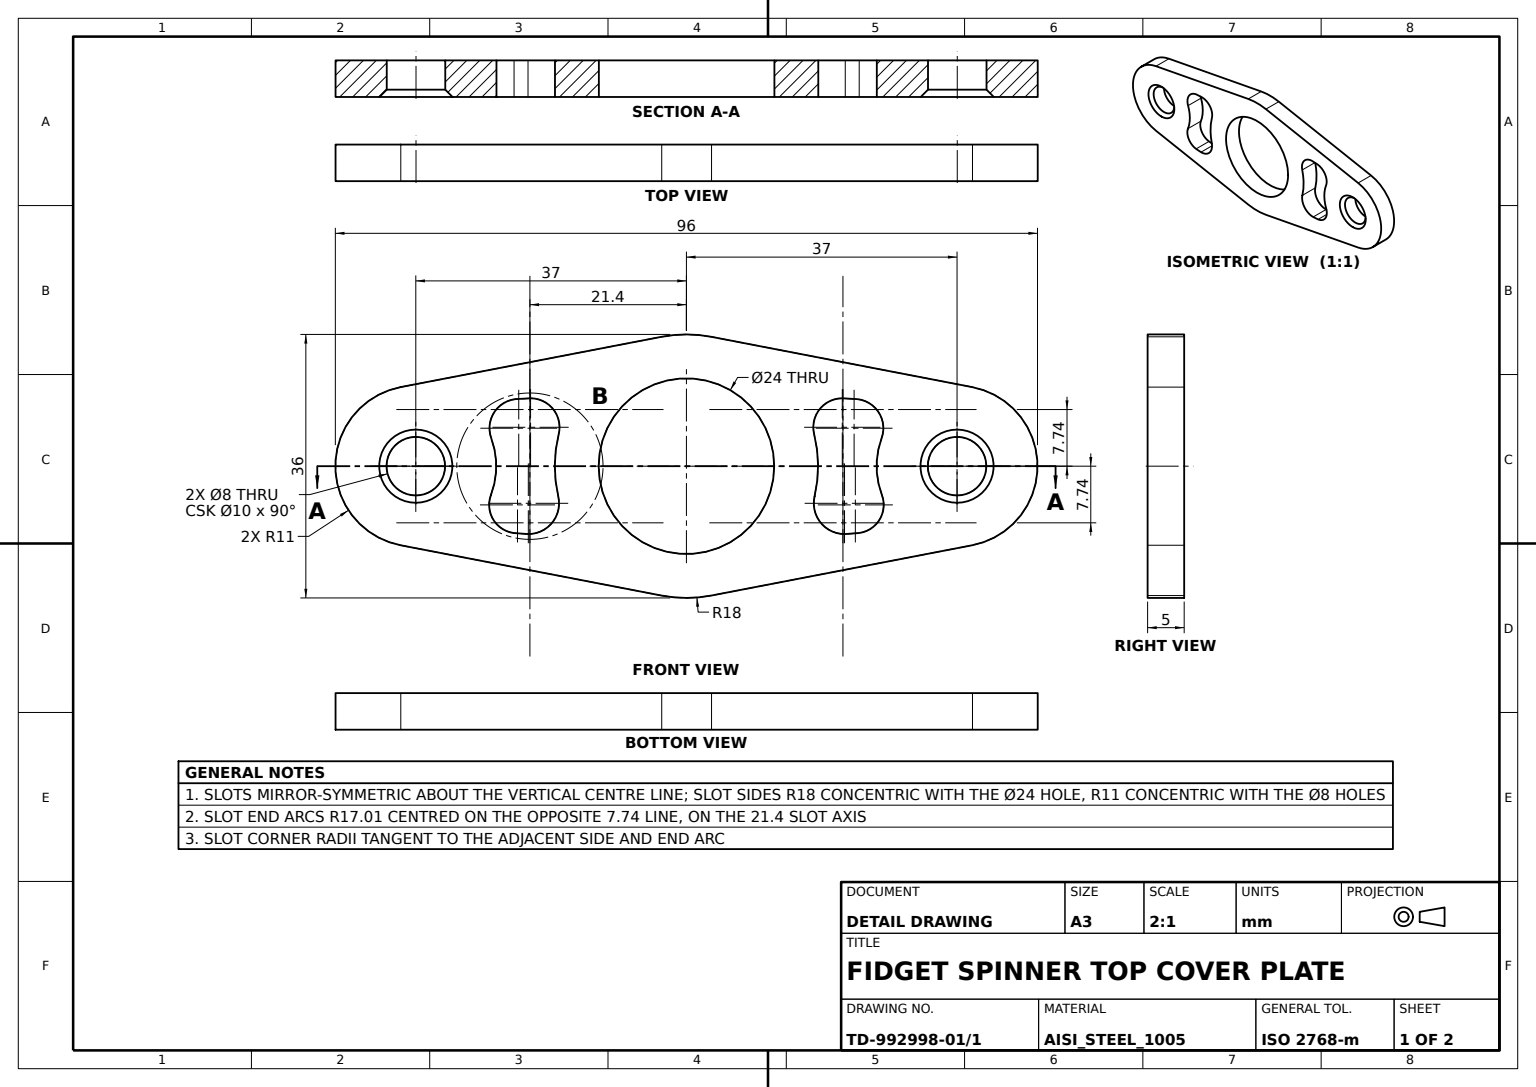
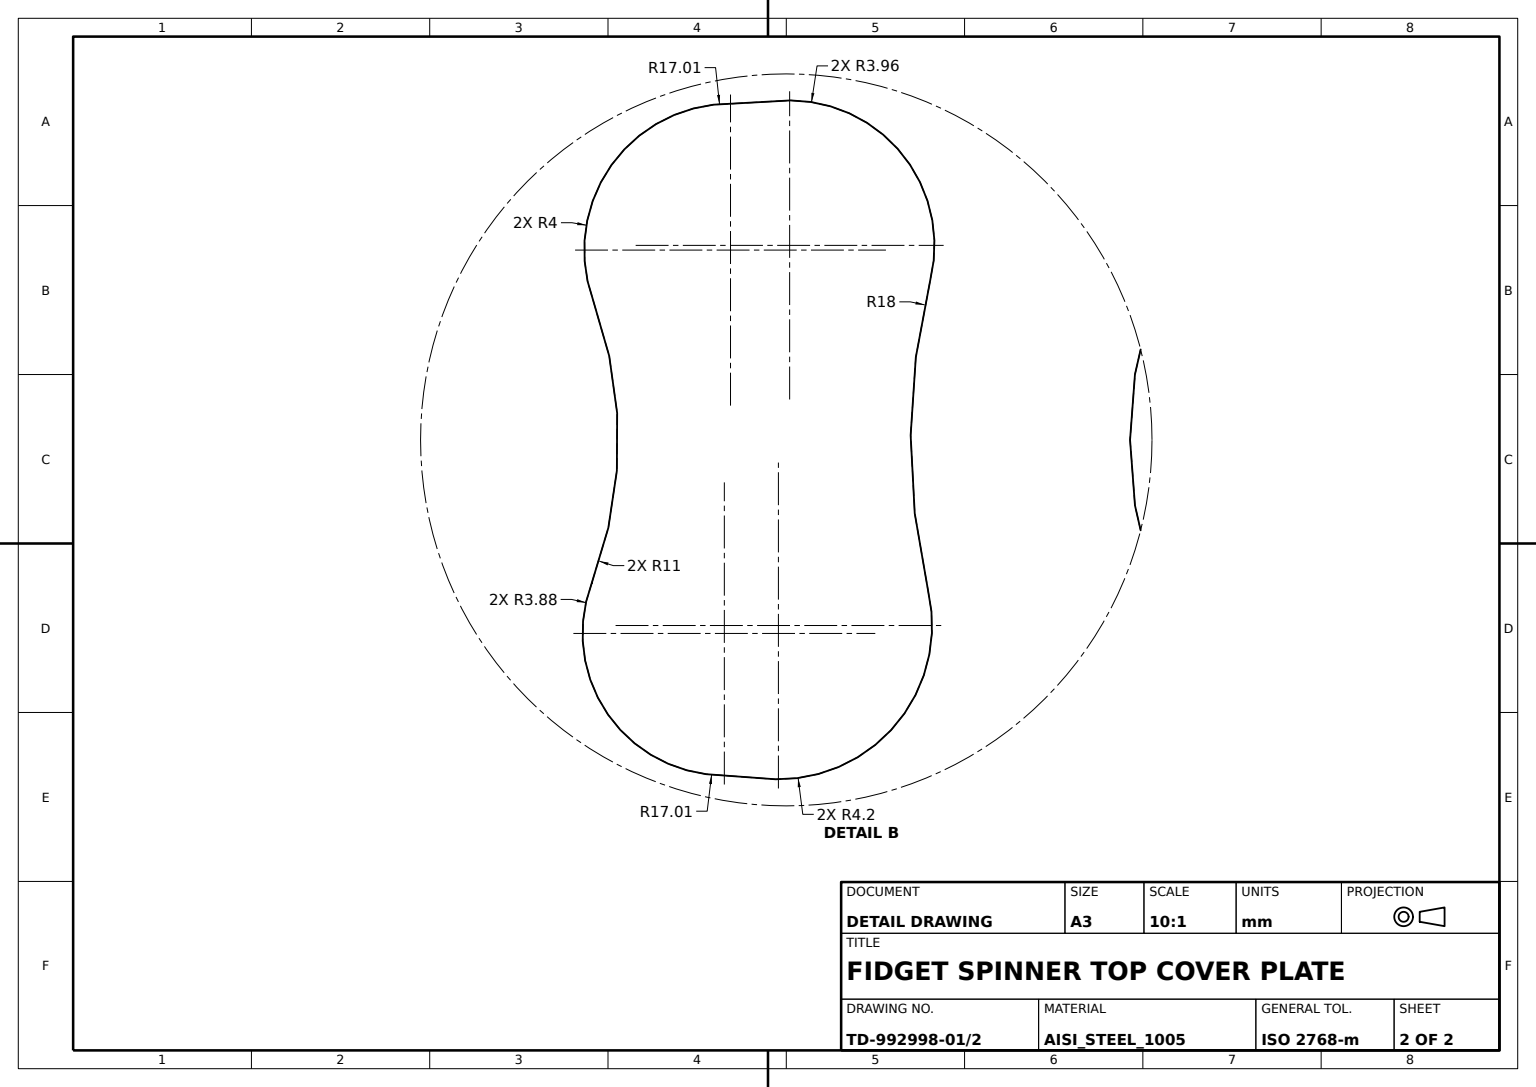
ISO-10303-21;
HEADER;
FILE_DESCRIPTION((''),'2;1');
FILE_NAME('','',(''),(''),'','','');
FILE_SCHEMA(('AUTOMOTIVE_DESIGN'));
ENDSEC;
DATA;
#1=APPLICATION_CONTEXT('');
#2=PRODUCT_CONTEXT('',#1,'mechanical');
#3=PRODUCT('','','',(#2));
#4=PRODUCT_DEFINITION_FORMATION('','',#3);
#5=PRODUCT_DEFINITION_CONTEXT('',#1,'design');
#6=PRODUCT_DEFINITION('','',#4,#5);
#7=PRODUCT_DEFINITION_SHAPE('','',#6);
#8=(LENGTH_UNIT()NAMED_UNIT(*)SI_UNIT(.MILLI.,.METRE.));
#9=(NAMED_UNIT(*)PLANE_ANGLE_UNIT()SI_UNIT($,.RADIAN.));
#10=(NAMED_UNIT(*)SI_UNIT($,.STERADIAN.)SOLID_ANGLE_UNIT());
#11=UNCERTAINTY_MEASURE_WITH_UNIT(LENGTH_MEASURE(0.005),#8,'distance_accuracy_value','');
#12=(GEOMETRIC_REPRESENTATION_CONTEXT(3)GLOBAL_UNCERTAINTY_ASSIGNED_CONTEXT((#11))GLOBAL_UNIT_ASSIGNED_CONTEXT((#8,#9,#10))REPRESENTATION_CONTEXT('',''));
#13=CARTESIAN_POINT('',(3.405405,-5.,17.674932));
#14=VERTEX_POINT('',#13);
#15=CARTESIAN_POINT('',(3.405405,0.,17.674932));
#16=VERTEX_POINT('',#15);
#17=DIRECTION('',(0.,1.,0.));
#18=VECTOR('',#17,1000.);
#19=LINE('',#13,#18);
#20=EDGE_CURVE('',#14,#16,#19,.T.);
#21=ORIENTED_EDGE('',*,*,#20,.T.);
#22=CARTESIAN_POINT('',(-3.405405,0.,17.674932));
#23=VERTEX_POINT('',#22);
#24=CARTESIAN_POINT('',(0.,0.,0.));
#25=DIRECTION('',(0.,-1.,0.));
#26=DIRECTION('',(1.,0.,0.));
#27=AXIS2_PLACEMENT_3D('',#24,#25,#26);
#28=CIRCLE('',#27,18.);
#29=EDGE_CURVE('',#16,#23,#28,.T.);
#30=ORIENTED_EDGE('',*,*,#29,.T.);
#31=CARTESIAN_POINT('',(-3.405405,-5.,17.674932));
#32=VERTEX_POINT('',#31);
#33=LINE('',#31,#18);
#34=EDGE_CURVE('',#32,#23,#33,.T.);
#35=ORIENTED_EDGE('',*,*,#34,.F.);
#36=CARTESIAN_POINT('',(0.,-5.,0.));
#37=AXIS2_PLACEMENT_3D('',#36,#25,#26);
#38=CIRCLE('',#37,18.);
#39=EDGE_CURVE('',#14,#32,#38,.T.);
#40=ORIENTED_EDGE('',*,*,#39,.F.);
#41=EDGE_LOOP('',(#21,#30,#35,#40));
#42=FACE_BOUND('',#41,.T.);
#43=DIRECTION('',(0.,0.,1.));
#44=AXIS2_PLACEMENT_3D('',#36,#17,#43);
#45=CYLINDRICAL_SURFACE('',#44,18.);
#46=ADVANCED_FACE('',(#42),#45,.T.);
#47=CARTESIAN_POINT('',(-33.,0.,0.));
#48=VERTEX_POINT('',#47);
#49=CARTESIAN_POINT('',(-37.,0.,0.));
#50=AXIS2_PLACEMENT_3D('',#49,#25,#26);
#51=CIRCLE('',#50,4.);
#52=EDGE_CURVE('',#48,#48,#51,.T.);
#53=ORIENTED_EDGE('',*,*,#52,.F.);
#54=EDGE_LOOP('',(#53));
#55=FACE_BOUND('',#54,.T.);
#56=CARTESIAN_POINT('',(-37.,-4.,-4.));
#57=VERTEX_POINT('',#56);
#58=CARTESIAN_POINT('',(-37.,-4.,0.));
#59=DIRECTION('',(0.,0.,-1.));
#60=AXIS2_PLACEMENT_3D('',#58,#25,#59);
#61=CIRCLE('',#60,4.);
#62=EDGE_CURVE('',#57,#57,#61,.T.);
#63=ORIENTED_EDGE('',*,*,#62,.T.);
#64=EDGE_LOOP('',(#63));
#65=FACE_BOUND('',#64,.T.);
#66=CARTESIAN_POINT('',(-37.,-5.,0.));
#67=AXIS2_PLACEMENT_3D('',#66,#17,#43);
#68=CYLINDRICAL_SURFACE('',#67,4.);
#69=ADVANCED_FACE('',(#55,#65),#68,.F.);
#70=CARTESIAN_POINT('',(39.081081,0.,10.801347));
#71=VERTEX_POINT('',#70);
#72=DIRECTION('',(-0.981940655,0.,0.189189189));
#73=VECTOR('',#72,1000.);
#74=LINE('',#70,#73);
#75=EDGE_CURVE('',#71,#16,#74,.T.);
#76=ORIENTED_EDGE('',*,*,#75,.T.);
#77=ORIENTED_EDGE('',*,*,#20,.F.);
#78=CARTESIAN_POINT('',(39.081081,-5.,10.801347));
#79=VERTEX_POINT('',#78);
#80=LINE('',#78,#73);
#81=EDGE_CURVE('',#79,#14,#80,.T.);
#82=ORIENTED_EDGE('',*,*,#81,.F.);
#83=LINE('',#78,#18);
#84=EDGE_CURVE('',#79,#71,#83,.T.);
#85=ORIENTED_EDGE('',*,*,#84,.T.);
#86=EDGE_LOOP('',(#76,#77,#82,#85));
#87=FACE_BOUND('',#86,.T.);
#88=DIRECTION('',(-0.189189189,0.,-0.981940655));
#89=AXIS2_PLACEMENT_3D('',#78,#88,#72);
#90=PLANE('',#89);
#91=ADVANCED_FACE('',(#87),#90,.F.);
#92=CARTESIAN_POINT('',(-21.686605,-5.,-9.273515));
#93=VERTEX_POINT('',#92);
#94=CARTESIAN_POINT('',(-21.686605,0.,-9.273515));
#95=VERTEX_POINT('',#94);
#96=LINE('',#92,#18);
#97=EDGE_CURVE('',#93,#95,#96,.T.);
#98=ORIENTED_EDGE('',*,*,#97,.T.);
#99=CARTESIAN_POINT('',(-23.59451,0.,-9.133621));
#100=VERTEX_POINT('',#99);
#101=CARTESIAN_POINT('',(-21.398386,0.,7.737492));
#102=AXIS2_PLACEMENT_3D('',#101,#17,#26);
#103=CIRCLE('',#102,17.013449);
#104=EDGE_CURVE('',#95,#100,#103,.T.);
#105=ORIENTED_EDGE('',*,*,#104,.T.);
#106=CARTESIAN_POINT('',(-23.59451,-5.,-9.133621));
#107=VERTEX_POINT('',#106);
#108=LINE('',#106,#18);
#109=EDGE_CURVE('',#107,#100,#108,.T.);
#110=ORIENTED_EDGE('',*,*,#109,.F.);
#111=CARTESIAN_POINT('',(-21.398386,-5.,7.737492));
#112=AXIS2_PLACEMENT_3D('',#111,#17,#26);
#113=CIRCLE('',#112,17.013449);
#114=EDGE_CURVE('',#93,#107,#113,.T.);
#115=ORIENTED_EDGE('',*,*,#114,.F.);
#116=EDGE_LOOP('',(#98,#105,#110,#115));
#117=FACE_BOUND('',#116,.T.);
#118=AXIS2_PLACEMENT_3D('',#111,#17,#43);
#119=CYLINDRICAL_SURFACE('',#118,17.013449);
#120=ADVANCED_FACE('',(#117),#119,.F.);
#121=CARTESIAN_POINT('',(-26.678365,-5.,3.803138));
#122=VERTEX_POINT('',#121);
#123=CARTESIAN_POINT('',(-26.678365,0.,3.803138));
#124=VERTEX_POINT('',#123);
#125=LINE('',#121,#18);
#126=EDGE_CURVE('',#122,#124,#125,.T.);
#127=ORIENTED_EDGE('',*,*,#126,.F.);
#128=CARTESIAN_POINT('',(-26.718391,-5.,-3.910053));
#129=VERTEX_POINT('',#128);
#130=AXIS2_PLACEMENT_3D('',#66,#25,#26);
#131=CIRCLE('',#130,11.);
#132=EDGE_CURVE('',#129,#122,#131,.T.);
#133=ORIENTED_EDGE('',*,*,#132,.F.);
#134=CARTESIAN_POINT('',(-26.718391,0.,-3.910053));
#135=VERTEX_POINT('',#134);
#136=LINE('',#128,#18);
#137=EDGE_CURVE('',#129,#135,#136,.T.);
#138=ORIENTED_EDGE('',*,*,#137,.T.);
#139=CIRCLE('',#50,11.);
#140=EDGE_CURVE('',#135,#124,#139,.T.);
#141=ORIENTED_EDGE('',*,*,#140,.T.);
#142=EDGE_LOOP('',(#127,#133,#138,#141));
#143=FACE_BOUND('',#142,.T.);
#144=CYLINDRICAL_SURFACE('',#67,11.);
#145=ADVANCED_FACE('',(#143),#144,.T.);
#146=ORIENTED_EDGE('',*,*,#84,.F.);
#147=CARTESIAN_POINT('',(39.081081,-5.,-10.801347));
#148=VERTEX_POINT('',#147);
#149=CARTESIAN_POINT('',(37.,-5.,0.));
#150=DIRECTION('',(-1.,0.,0.));
#151=AXIS2_PLACEMENT_3D('',#149,#25,#150);
#152=CIRCLE('',#151,11.);
#153=EDGE_CURVE('',#148,#79,#152,.T.);
#154=ORIENTED_EDGE('',*,*,#153,.F.);
#155=CARTESIAN_POINT('',(39.081081,0.,-10.801347));
#156=VERTEX_POINT('',#155);
#157=LINE('',#147,#18);
#158=EDGE_CURVE('',#148,#156,#157,.T.);
#159=ORIENTED_EDGE('',*,*,#158,.T.);
#160=CARTESIAN_POINT('',(37.,0.,0.));
#161=AXIS2_PLACEMENT_3D('',#160,#25,#150);
#162=CIRCLE('',#161,11.);
#163=EDGE_CURVE('',#156,#71,#162,.T.);
#164=ORIENTED_EDGE('',*,*,#163,.T.);
#165=EDGE_LOOP('',(#146,#154,#159,#164));
#166=FACE_BOUND('',#165,.T.);
#167=AXIS2_PLACEMENT_3D('',#149,#17,#43);
#168=CYLINDRICAL_SURFACE('',#167,11.);
#169=ADVANCED_FACE('',(#166),#168,.T.);
#170=CARTESIAN_POINT('',(26.718391,-5.,-3.910053));
#171=VERTEX_POINT('',#170);
#172=CARTESIAN_POINT('',(26.718391,0.,-3.910053));
#173=VERTEX_POINT('',#172);
#174=LINE('',#170,#18);
#175=EDGE_CURVE('',#171,#173,#174,.T.);
#176=ORIENTED_EDGE('',*,*,#175,.F.);
#177=CARTESIAN_POINT('',(26.678365,-5.,3.803138));
#178=VERTEX_POINT('',#177);
#179=EDGE_CURVE('',#178,#171,#152,.T.);
#180=ORIENTED_EDGE('',*,*,#179,.F.);
#181=CARTESIAN_POINT('',(26.678365,0.,3.803138));
#182=VERTEX_POINT('',#181);
#183=LINE('',#177,#18);
#184=EDGE_CURVE('',#178,#182,#183,.T.);
#185=ORIENTED_EDGE('',*,*,#184,.T.);
#186=EDGE_CURVE('',#182,#173,#162,.T.);
#187=ORIENTED_EDGE('',*,*,#186,.T.);
#188=EDGE_LOOP('',(#176,#180,#185,#187));
#189=FACE_BOUND('',#188,.T.);
#190=ADVANCED_FACE('',(#189),#168,.T.);
#191=CARTESIAN_POINT('',(37.,-4.,-4.));
#192=VERTEX_POINT('',#191);
#193=CARTESIAN_POINT('',(37.,-4.,0.));
#194=AXIS2_PLACEMENT_3D('',#193,#25,#59);
#195=CIRCLE('',#194,4.);
#196=EDGE_CURVE('',#192,#192,#195,.T.);
#197=ORIENTED_EDGE('',*,*,#196,.T.);
#198=EDGE_LOOP('',(#197));
#199=FACE_BOUND('',#198,.T.);
#200=CARTESIAN_POINT('',(33.,0.,0.));
#201=VERTEX_POINT('',#200);
#202=AXIS2_PLACEMENT_3D('',#160,#17,#150);
#203=CIRCLE('',#202,4.);
#204=EDGE_CURVE('',#201,#201,#203,.T.);
#205=ORIENTED_EDGE('',*,*,#204,.T.);
#206=EDGE_LOOP('',(#205));
#207=FACE_BOUND('',#206,.T.);
#208=CYLINDRICAL_SURFACE('',#167,4.);
#209=ADVANCED_FACE('',(#199,#207),#208,.F.);
#210=CARTESIAN_POINT('',(23.394299,-5.,9.158477));
#211=VERTEX_POINT('',#210);
#212=CARTESIAN_POINT('',(23.394299,0.,9.158477));
#213=VERTEX_POINT('',#212);
#214=LINE('',#210,#18);
#215=EDGE_CURVE('',#211,#213,#214,.T.);
#216=ORIENTED_EDGE('',*,*,#215,.F.);
#217=CARTESIAN_POINT('',(21.280547,-5.,9.275548));
#218=VERTEX_POINT('',#217);
#219=CARTESIAN_POINT('',(21.398386,-5.,-7.737492));
#220=AXIS2_PLACEMENT_3D('',#219,#17,#150);
#221=CIRCLE('',#220,17.013449);
#222=EDGE_CURVE('',#218,#211,#221,.T.);
#223=ORIENTED_EDGE('',*,*,#222,.F.);
#224=CARTESIAN_POINT('',(21.280547,0.,9.275548));
#225=VERTEX_POINT('',#224);
#226=LINE('',#217,#18);
#227=EDGE_CURVE('',#218,#225,#226,.T.);
#228=ORIENTED_EDGE('',*,*,#227,.T.);
#229=CARTESIAN_POINT('',(21.398386,0.,-7.737492));
#230=AXIS2_PLACEMENT_3D('',#229,#17,#150);
#231=CIRCLE('',#230,17.013449);
#232=EDGE_CURVE('',#225,#213,#231,.T.);
#233=ORIENTED_EDGE('',*,*,#232,.T.);
#234=EDGE_LOOP('',(#216,#223,#228,#233));
#235=FACE_BOUND('',#234,.T.);
#236=AXIS2_PLACEMENT_3D('',#219,#17,#43);
#237=CYLINDRICAL_SURFACE('',#236,17.013449);
#238=ADVANCED_FACE('',(#235),#237,.F.);
#239=CARTESIAN_POINT('',(-21.280547,-5.,9.275548));
#240=VERTEX_POINT('',#239);
#241=CARTESIAN_POINT('',(-21.280547,0.,9.275548));
#242=VERTEX_POINT('',#241);
#243=LINE('',#239,#18);
#244=EDGE_CURVE('',#240,#242,#243,.T.);
#245=ORIENTED_EDGE('',*,*,#244,.F.);
#246=CARTESIAN_POINT('',(-23.394299,-5.,9.158477));
#247=VERTEX_POINT('',#246);
#248=CARTESIAN_POINT('',(-21.398386,-5.,-7.737492));
#249=AXIS2_PLACEMENT_3D('',#248,#17,#26);
#250=CIRCLE('',#249,17.013449);
#251=EDGE_CURVE('',#247,#240,#250,.T.);
#252=ORIENTED_EDGE('',*,*,#251,.F.);
#253=CARTESIAN_POINT('',(-23.394299,0.,9.158477));
#254=VERTEX_POINT('',#253);
#255=LINE('',#246,#18);
#256=EDGE_CURVE('',#247,#254,#255,.T.);
#257=ORIENTED_EDGE('',*,*,#256,.T.);
#258=CARTESIAN_POINT('',(-21.398386,0.,-7.737492));
#259=AXIS2_PLACEMENT_3D('',#258,#17,#26);
#260=CIRCLE('',#259,17.013449);
#261=EDGE_CURVE('',#254,#242,#260,.T.);
#262=ORIENTED_EDGE('',*,*,#261,.T.);
#263=EDGE_LOOP('',(#245,#252,#257,#262));
#264=FACE_BOUND('',#263,.T.);
#265=AXIS2_PLACEMENT_3D('',#248,#17,#43);
#266=CYLINDRICAL_SURFACE('',#265,17.013449);
#267=ADVANCED_FACE('',(#264),#266,.F.);
#268=CARTESIAN_POINT('',(-17.464909,-5.,4.356254));
#269=VERTEX_POINT('',#268);
#270=CARTESIAN_POINT('',(-17.464909,0.,4.356254));
#271=VERTEX_POINT('',#270);
#272=LINE('',#268,#18);
#273=EDGE_CURVE('',#269,#271,#272,.T.);
#274=ORIENTED_EDGE('',*,*,#273,.F.);
#275=CARTESIAN_POINT('',(-21.307981,-5.,5.314827));
#276=AXIS2_PLACEMENT_3D('',#275,#17,#26);
#277=CIRCLE('',#276,3.960816);
#278=EDGE_CURVE('',#240,#269,#277,.T.);
#279=ORIENTED_EDGE('',*,*,#278,.F.);
#280=ORIENTED_EDGE('',*,*,#244,.T.);
#281=CARTESIAN_POINT('',(-21.307981,0.,5.314827));
#282=AXIS2_PLACEMENT_3D('',#281,#17,#26);
#283=CIRCLE('',#282,3.960816);
#284=EDGE_CURVE('',#242,#271,#283,.T.);
#285=ORIENTED_EDGE('',*,*,#284,.T.);
#286=EDGE_LOOP('',(#274,#279,#280,#285));
#287=FACE_BOUND('',#286,.T.);
#288=AXIS2_PLACEMENT_3D('',#275,#17,#43);
#289=CYLINDRICAL_SURFACE('',#288,3.960816);
#290=ADVANCED_FACE('',(#287),#289,.F.);
#291=CARTESIAN_POINT('',(17.464909,-5.,4.356254));
#292=VERTEX_POINT('',#291);
#293=CARTESIAN_POINT('',(17.464909,0.,4.356254));
#294=VERTEX_POINT('',#293);
#295=LINE('',#291,#18);
#296=EDGE_CURVE('',#292,#294,#295,.T.);
#297=ORIENTED_EDGE('',*,*,#296,.F.);
#298=CARTESIAN_POINT('',(17.52409,-5.,-4.111725));
#299=VERTEX_POINT('',#298);
#300=AXIS2_PLACEMENT_3D('',#36,#25,#150);
#301=CIRCLE('',#300,18.);
#302=EDGE_CURVE('',#299,#292,#301,.T.);
#303=ORIENTED_EDGE('',*,*,#302,.F.);
#304=CARTESIAN_POINT('',(17.52409,0.,-4.111725));
#305=VERTEX_POINT('',#304);
#306=LINE('',#298,#18);
#307=EDGE_CURVE('',#299,#305,#306,.T.);
#308=ORIENTED_EDGE('',*,*,#307,.T.);
#309=AXIS2_PLACEMENT_3D('',#24,#25,#150);
#310=CIRCLE('',#309,18.);
#311=EDGE_CURVE('',#305,#294,#310,.T.);
#312=ORIENTED_EDGE('',*,*,#311,.T.);
#313=EDGE_LOOP('',(#297,#303,#308,#312));
#314=FACE_BOUND('',#313,.T.);
#315=ADVANCED_FACE('',(#314),#45,.T.);
#316=CARTESIAN_POINT('',(-37.,-5.,-5.));
#317=VERTEX_POINT('',#316);
#318=AXIS2_PLACEMENT_3D('',#66,#25,#59);
#319=CIRCLE('',#318,5.);
#320=EDGE_CURVE('',#317,#317,#319,.F.);
#321=ORIENTED_EDGE('',*,*,#320,.F.);
#322=EDGE_LOOP('',(#321));
#323=FACE_BOUND('',#322,.T.);
#324=ORIENTED_EDGE('',*,*,#62,.F.);
#325=EDGE_LOOP('',(#324));
#326=FACE_BOUND('',#325,.T.);
#327=CONICAL_SURFACE('',#60,4.,0.785398163);
#328=ADVANCED_FACE('',(#323,#326),#327,.F.);
#329=CARTESIAN_POINT('',(22.925044,-5.,5.186097));
#330=AXIS2_PLACEMENT_3D('',#329,#17,#150);
#331=CIRCLE('',#330,4.);
#332=EDGE_CURVE('',#211,#178,#331,.T.);
#333=ORIENTED_EDGE('',*,*,#332,.F.);
#334=ORIENTED_EDGE('',*,*,#215,.T.);
#335=CARTESIAN_POINT('',(22.925044,0.,5.186097));
#336=AXIS2_PLACEMENT_3D('',#335,#17,#150);
#337=CIRCLE('',#336,4.);
#338=EDGE_CURVE('',#213,#182,#337,.T.);
#339=ORIENTED_EDGE('',*,*,#338,.T.);
#340=ORIENTED_EDGE('',*,*,#184,.F.);
#341=EDGE_LOOP('',(#333,#334,#339,#340));
#342=FACE_BOUND('',#341,.T.);
#343=AXIS2_PLACEMENT_3D('',#329,#17,#43);
#344=CYLINDRICAL_SURFACE('',#343,4.);
#345=ADVANCED_FACE('',(#342),#344,.F.);
#346=CARTESIAN_POINT('',(-39.081081,-5.,10.801347));
#347=VERTEX_POINT('',#346);
#348=CARTESIAN_POINT('',(-39.081081,-5.,-10.801347));
#349=VERTEX_POINT('',#348);
#350=EDGE_CURVE('',#347,#349,#131,.T.);
#351=ORIENTED_EDGE('',*,*,#350,.F.);
#352=CARTESIAN_POINT('',(-39.081081,0.,10.801347));
#353=VERTEX_POINT('',#352);
#354=LINE('',#346,#18);
#355=EDGE_CURVE('',#347,#353,#354,.T.);
#356=ORIENTED_EDGE('',*,*,#355,.T.);
#357=CARTESIAN_POINT('',(-39.081081,0.,-10.801347));
#358=VERTEX_POINT('',#357);
#359=EDGE_CURVE('',#353,#358,#139,.T.);
#360=ORIENTED_EDGE('',*,*,#359,.T.);
#361=LINE('',#348,#18);
#362=EDGE_CURVE('',#349,#358,#361,.T.);
#363=ORIENTED_EDGE('',*,*,#362,.F.);
#364=EDGE_LOOP('',(#351,#356,#360,#363));
#365=FACE_BOUND('',#364,.T.);
#366=ADVANCED_FACE('',(#365),#144,.T.);
#367=CARTESIAN_POINT('',(23.59451,0.,-9.133621));
#368=VERTEX_POINT('',#367);
#369=CARTESIAN_POINT('',(21.686605,0.,-9.273515));
#370=VERTEX_POINT('',#369);
#371=CARTESIAN_POINT('',(21.398386,0.,7.737492));
#372=AXIS2_PLACEMENT_3D('',#371,#17,#150);
#373=CIRCLE('',#372,17.013449);
#374=EDGE_CURVE('',#368,#370,#373,.T.);
#375=ORIENTED_EDGE('',*,*,#374,.T.);
#376=CARTESIAN_POINT('',(21.686605,-5.,-9.273515));
#377=VERTEX_POINT('',#376);
#378=LINE('',#376,#18);
#379=EDGE_CURVE('',#377,#370,#378,.T.);
#380=ORIENTED_EDGE('',*,*,#379,.F.);
#381=CARTESIAN_POINT('',(23.59451,-5.,-9.133621));
#382=VERTEX_POINT('',#381);
#383=CARTESIAN_POINT('',(21.398386,-5.,7.737492));
#384=AXIS2_PLACEMENT_3D('',#383,#17,#150);
#385=CIRCLE('',#384,17.013449);
#386=EDGE_CURVE('',#382,#377,#385,.T.);
#387=ORIENTED_EDGE('',*,*,#386,.F.);
#388=LINE('',#381,#18);
#389=EDGE_CURVE('',#382,#368,#388,.T.);
#390=ORIENTED_EDGE('',*,*,#389,.T.);
#391=EDGE_LOOP('',(#375,#380,#387,#390));
#392=FACE_BOUND('',#391,.T.);
#393=AXIS2_PLACEMENT_3D('',#383,#17,#43);
#394=CYLINDRICAL_SURFACE('',#393,17.013449);
#395=ADVANCED_FACE('',(#392),#394,.F.);
#396=ORIENTED_EDGE('',*,*,#175,.T.);
#397=CARTESIAN_POINT('',(23.093976,0.,-5.288403));
#398=AXIS2_PLACEMENT_3D('',#397,#17,#150);
#399=CIRCLE('',#398,3.877658);
#400=EDGE_CURVE('',#173,#368,#399,.T.);
#401=ORIENTED_EDGE('',*,*,#400,.T.);
#402=ORIENTED_EDGE('',*,*,#389,.F.);
#403=CARTESIAN_POINT('',(23.093976,-5.,-5.288403));
#404=AXIS2_PLACEMENT_3D('',#403,#17,#150);
#405=CIRCLE('',#404,3.877658);
#406=EDGE_CURVE('',#171,#382,#405,.T.);
#407=ORIENTED_EDGE('',*,*,#406,.F.);
#408=EDGE_LOOP('',(#396,#401,#402,#407));
#409=FACE_BOUND('',#408,.T.);
#410=AXIS2_PLACEMENT_3D('',#403,#17,#43);
#411=CYLINDRICAL_SURFACE('',#410,3.877658);
#412=ADVANCED_FACE('',(#409),#411,.F.);
#413=CARTESIAN_POINT('',(-3.405405,-5.,-17.674932));
#414=VERTEX_POINT('',#413);
#415=CARTESIAN_POINT('',(3.405405,-5.,-17.674932));
#416=VERTEX_POINT('',#415);
#417=EDGE_CURVE('',#414,#416,#38,.T.);
#418=ORIENTED_EDGE('',*,*,#417,.F.);
#419=CARTESIAN_POINT('',(-3.405405,0.,-17.674932));
#420=VERTEX_POINT('',#419);
#421=LINE('',#413,#18);
#422=EDGE_CURVE('',#414,#420,#421,.T.);
#423=ORIENTED_EDGE('',*,*,#422,.T.);
#424=CARTESIAN_POINT('',(3.405405,0.,-17.674932));
#425=VERTEX_POINT('',#424);
#426=EDGE_CURVE('',#420,#425,#28,.T.);
#427=ORIENTED_EDGE('',*,*,#426,.T.);
#428=LINE('',#415,#18);
#429=EDGE_CURVE('',#416,#425,#428,.T.);
#430=ORIENTED_EDGE('',*,*,#429,.F.);
#431=EDGE_LOOP('',(#418,#423,#427,#430));
#432=FACE_BOUND('',#431,.T.);
#433=ADVANCED_FACE('',(#432),#45,.T.);
#434=ORIENTED_EDGE('',*,*,#196,.F.);
#435=EDGE_LOOP('',(#434));
#436=FACE_BOUND('',#435,.T.);
#437=CARTESIAN_POINT('',(37.,-5.,-5.));
#438=VERTEX_POINT('',#437);
#439=AXIS2_PLACEMENT_3D('',#149,#25,#59);
#440=CIRCLE('',#439,5.);
#441=EDGE_CURVE('',#438,#438,#440,.F.);
#442=ORIENTED_EDGE('',*,*,#441,.F.);
#443=EDGE_LOOP('',(#442));
#444=FACE_BOUND('',#443,.T.);
#445=CONICAL_SURFACE('',#439,5.,0.785398163);
#446=ADVANCED_FACE('',(#436,#444),#445,.F.);
#447=CARTESIAN_POINT('',(-23.093976,0.,-5.288403));
#448=AXIS2_PLACEMENT_3D('',#447,#17,#26);
#449=CIRCLE('',#448,3.877658);
#450=EDGE_CURVE('',#100,#135,#449,.T.);
#451=ORIENTED_EDGE('',*,*,#450,.T.);
#452=ORIENTED_EDGE('',*,*,#137,.F.);
#453=CARTESIAN_POINT('',(-23.093976,-5.,-5.288403));
#454=AXIS2_PLACEMENT_3D('',#453,#17,#26);
#455=CIRCLE('',#454,3.877658);
#456=EDGE_CURVE('',#107,#129,#455,.T.);
#457=ORIENTED_EDGE('',*,*,#456,.F.);
#458=ORIENTED_EDGE('',*,*,#109,.T.);
#459=EDGE_LOOP('',(#451,#452,#457,#458));
#460=FACE_BOUND('',#459,.T.);
#461=AXIS2_PLACEMENT_3D('',#453,#17,#43);
#462=CYLINDRICAL_SURFACE('',#461,3.877658);
#463=ADVANCED_FACE('',(#460),#462,.F.);
#464=DIRECTION('',(-0.981940655,0.,-0.189189189));
#465=VECTOR('',#464,1000.);
#466=LINE('',#31,#465);
#467=EDGE_CURVE('',#32,#347,#466,.T.);
#468=ORIENTED_EDGE('',*,*,#467,.F.);
#469=ORIENTED_EDGE('',*,*,#34,.T.);
#470=LINE('',#22,#465);
#471=EDGE_CURVE('',#23,#353,#470,.T.);
#472=ORIENTED_EDGE('',*,*,#471,.T.);
#473=ORIENTED_EDGE('',*,*,#355,.F.);
#474=EDGE_LOOP('',(#468,#469,#472,#473));
#475=FACE_BOUND('',#474,.T.);
#476=DIRECTION('',(0.189189189,0.,-0.981940655));
#477=AXIS2_PLACEMENT_3D('',#31,#476,#464);
#478=PLANE('',#477);
#479=ADVANCED_FACE('',(#475),#478,.F.);
#480=CARTESIAN_POINT('',(-22.925044,-5.,5.186097));
#481=AXIS2_PLACEMENT_3D('',#480,#17,#26);
#482=CIRCLE('',#481,4.);
#483=EDGE_CURVE('',#122,#247,#482,.T.);
#484=ORIENTED_EDGE('',*,*,#483,.F.);
#485=ORIENTED_EDGE('',*,*,#126,.T.);
#486=CARTESIAN_POINT('',(-22.925044,0.,5.186097));
#487=AXIS2_PLACEMENT_3D('',#486,#17,#26);
#488=CIRCLE('',#487,4.);
#489=EDGE_CURVE('',#124,#254,#488,.T.);
#490=ORIENTED_EDGE('',*,*,#489,.T.);
#491=ORIENTED_EDGE('',*,*,#256,.F.);
#492=EDGE_LOOP('',(#484,#485,#490,#491));
#493=FACE_BOUND('',#492,.T.);
#494=AXIS2_PLACEMENT_3D('',#480,#17,#43);
#495=CYLINDRICAL_SURFACE('',#494,4.);
#496=ADVANCED_FACE('',(#493),#495,.F.);
#497=CARTESIAN_POINT('',(12.,0.,0.));
#498=VERTEX_POINT('',#497);
#499=CIRCLE('',#27,12.);
#500=EDGE_CURVE('',#498,#498,#499,.T.);
#501=ORIENTED_EDGE('',*,*,#500,.T.);
#502=EDGE_LOOP('',(#501));
#503=FACE_BOUND('',#502,.T.);
#504=ORIENTED_EDGE('',*,*,#311,.F.);
#505=CARTESIAN_POINT('',(21.615413,0.,-5.071684));
#506=AXIS2_PLACEMENT_3D('',#505,#17,#150);
#507=CIRCLE('',#506,4.202434);
#508=EDGE_CURVE('',#370,#305,#507,.T.);
#509=ORIENTED_EDGE('',*,*,#508,.F.);
#510=ORIENTED_EDGE('',*,*,#374,.F.);
#511=ORIENTED_EDGE('',*,*,#400,.F.);
#512=ORIENTED_EDGE('',*,*,#186,.F.);
#513=ORIENTED_EDGE('',*,*,#338,.F.);
#514=ORIENTED_EDGE('',*,*,#232,.F.);
#515=CARTESIAN_POINT('',(21.307981,0.,5.314827));
#516=AXIS2_PLACEMENT_3D('',#515,#17,#150);
#517=CIRCLE('',#516,3.960816);
#518=EDGE_CURVE('',#294,#225,#517,.T.);
#519=ORIENTED_EDGE('',*,*,#518,.F.);
#520=EDGE_LOOP('',(#504,#509,#510,#511,#512,#513,#514,#519));
#521=FACE_BOUND('',#520,.T.);
#522=ORIENTED_EDGE('',*,*,#52,.T.);
#523=EDGE_LOOP('',(#522));
#524=FACE_BOUND('',#523,.T.);
#525=ORIENTED_EDGE('',*,*,#359,.F.);
#526=ORIENTED_EDGE('',*,*,#471,.F.);
#527=ORIENTED_EDGE('',*,*,#29,.F.);
#528=ORIENTED_EDGE('',*,*,#75,.F.);
#529=ORIENTED_EDGE('',*,*,#163,.F.);
#530=DIRECTION('',(0.981940655,0.,0.189189189));
#531=VECTOR('',#530,1000.);
#532=LINE('',#424,#531);
#533=EDGE_CURVE('',#425,#156,#532,.T.);
#534=ORIENTED_EDGE('',*,*,#533,.F.);
#535=ORIENTED_EDGE('',*,*,#426,.F.);
#536=DIRECTION('',(0.981940655,0.,-0.189189189));
#537=VECTOR('',#536,1000.);
#538=LINE('',#357,#537);
#539=EDGE_CURVE('',#358,#420,#538,.T.);
#540=ORIENTED_EDGE('',*,*,#539,.F.);
#541=EDGE_LOOP('',(#525,#526,#527,#528,#529,#534,#535,#540));
#542=FACE_BOUND('',#541,.T.);
#543=ORIENTED_EDGE('',*,*,#204,.F.);
#544=EDGE_LOOP('',(#543));
#545=FACE_BOUND('',#544,.T.);
#546=ORIENTED_EDGE('',*,*,#140,.F.);
#547=ORIENTED_EDGE('',*,*,#450,.F.);
#548=ORIENTED_EDGE('',*,*,#104,.F.);
#549=CARTESIAN_POINT('',(-17.52409,0.,-4.111725));
#550=VERTEX_POINT('',#549);
#551=CARTESIAN_POINT('',(-21.615413,0.,-5.071684));
#552=AXIS2_PLACEMENT_3D('',#551,#17,#26);
#553=CIRCLE('',#552,4.202434);
#554=EDGE_CURVE('',#550,#95,#553,.T.);
#555=ORIENTED_EDGE('',*,*,#554,.F.);
#556=EDGE_CURVE('',#271,#550,#28,.T.);
#557=ORIENTED_EDGE('',*,*,#556,.F.);
#558=ORIENTED_EDGE('',*,*,#284,.F.);
#559=ORIENTED_EDGE('',*,*,#261,.F.);
#560=ORIENTED_EDGE('',*,*,#489,.F.);
#561=EDGE_LOOP('',(#546,#547,#548,#555,#557,#558,#559,#560));
#562=FACE_BOUND('',#561,.T.);
#563=AXIS2_PLACEMENT_3D('',#49,#25,#59);
#564=PLANE('',#563);
#565=ADVANCED_FACE('',(#503,#521,#524,#542,#545,#562),#564,.F.);
#566=ORIENTED_EDGE('',*,*,#429,.T.);
#567=ORIENTED_EDGE('',*,*,#533,.T.);
#568=ORIENTED_EDGE('',*,*,#158,.F.);
#569=LINE('',#415,#531);
#570=EDGE_CURVE('',#416,#148,#569,.T.);
#571=ORIENTED_EDGE('',*,*,#570,.F.);
#572=EDGE_LOOP('',(#566,#567,#568,#571));
#573=FACE_BOUND('',#572,.T.);
#574=DIRECTION('',(-0.189189189,0.,0.981940655));
#575=AXIS2_PLACEMENT_3D('',#415,#574,#530);
#576=PLANE('',#575);
#577=ADVANCED_FACE('',(#573),#576,.F.);
#578=ORIENTED_EDGE('',*,*,#518,.T.);
#579=ORIENTED_EDGE('',*,*,#227,.F.);
#580=CARTESIAN_POINT('',(21.307981,-5.,5.314827));
#581=AXIS2_PLACEMENT_3D('',#580,#17,#150);
#582=CIRCLE('',#581,3.960816);
#583=EDGE_CURVE('',#292,#218,#582,.T.);
#584=ORIENTED_EDGE('',*,*,#583,.F.);
#585=ORIENTED_EDGE('',*,*,#296,.T.);
#586=EDGE_LOOP('',(#578,#579,#584,#585));
#587=FACE_BOUND('',#586,.T.);
#588=AXIS2_PLACEMENT_3D('',#580,#17,#43);
#589=CYLINDRICAL_SURFACE('',#588,3.960816);
#590=ADVANCED_FACE('',(#587),#589,.F.);
#591=ORIENTED_EDGE('',*,*,#500,.F.);
#592=EDGE_LOOP('',(#591));
#593=FACE_BOUND('',#592,.T.);
#594=CARTESIAN_POINT('',(12.,-5.,0.));
#595=VERTEX_POINT('',#594);
#596=CIRCLE('',#37,12.);
#597=EDGE_CURVE('',#595,#595,#596,.T.);
#598=ORIENTED_EDGE('',*,*,#597,.T.);
#599=EDGE_LOOP('',(#598));
#600=FACE_BOUND('',#599,.T.);
#601=CYLINDRICAL_SURFACE('',#44,12.);
#602=ADVANCED_FACE('',(#593,#600),#601,.F.);
#603=ORIENTED_EDGE('',*,*,#251,.T.);
#604=ORIENTED_EDGE('',*,*,#278,.T.);
#605=CARTESIAN_POINT('',(-17.52409,-5.,-4.111725));
#606=VERTEX_POINT('',#605);
#607=EDGE_CURVE('',#269,#606,#38,.T.);
#608=ORIENTED_EDGE('',*,*,#607,.T.);
#609=CARTESIAN_POINT('',(-21.615413,-5.,-5.071684));
#610=AXIS2_PLACEMENT_3D('',#609,#17,#26);
#611=CIRCLE('',#610,4.202434);
#612=EDGE_CURVE('',#606,#93,#611,.T.);
#613=ORIENTED_EDGE('',*,*,#612,.T.);
#614=ORIENTED_EDGE('',*,*,#114,.T.);
#615=ORIENTED_EDGE('',*,*,#456,.T.);
#616=ORIENTED_EDGE('',*,*,#132,.T.);
#617=ORIENTED_EDGE('',*,*,#483,.T.);
#618=EDGE_LOOP('',(#603,#604,#608,#613,#614,#615,#616,#617));
#619=FACE_BOUND('',#618,.T.);
#620=ORIENTED_EDGE('',*,*,#597,.F.);
#621=EDGE_LOOP('',(#620));
#622=FACE_BOUND('',#621,.T.);
#623=ORIENTED_EDGE('',*,*,#153,.T.);
#624=ORIENTED_EDGE('',*,*,#81,.T.);
#625=ORIENTED_EDGE('',*,*,#39,.T.);
#626=ORIENTED_EDGE('',*,*,#467,.T.);
#627=ORIENTED_EDGE('',*,*,#350,.T.);
#628=LINE('',#348,#537);
#629=EDGE_CURVE('',#349,#414,#628,.T.);
#630=ORIENTED_EDGE('',*,*,#629,.T.);
#631=ORIENTED_EDGE('',*,*,#417,.T.);
#632=ORIENTED_EDGE('',*,*,#570,.T.);
#633=EDGE_LOOP('',(#623,#624,#625,#626,#627,#630,#631,#632));
#634=FACE_BOUND('',#633,.T.);
#635=ORIENTED_EDGE('',*,*,#441,.T.);
#636=EDGE_LOOP('',(#635));
#637=FACE_BOUND('',#636,.T.);
#638=ORIENTED_EDGE('',*,*,#302,.T.);
#639=ORIENTED_EDGE('',*,*,#583,.T.);
#640=ORIENTED_EDGE('',*,*,#222,.T.);
#641=ORIENTED_EDGE('',*,*,#332,.T.);
#642=ORIENTED_EDGE('',*,*,#179,.T.);
#643=ORIENTED_EDGE('',*,*,#406,.T.);
#644=ORIENTED_EDGE('',*,*,#386,.T.);
#645=CARTESIAN_POINT('',(21.615413,-5.,-5.071684));
#646=AXIS2_PLACEMENT_3D('',#645,#17,#150);
#647=CIRCLE('',#646,4.202434);
#648=EDGE_CURVE('',#377,#299,#647,.T.);
#649=ORIENTED_EDGE('',*,*,#648,.T.);
#650=EDGE_LOOP('',(#638,#639,#640,#641,#642,#643,#644,#649));
#651=FACE_BOUND('',#650,.T.);
#652=ORIENTED_EDGE('',*,*,#320,.T.);
#653=EDGE_LOOP('',(#652));
#654=FACE_BOUND('',#653,.T.);
#655=PLANE('',#318);
#656=ADVANCED_FACE('',(#619,#622,#634,#637,#651,#654),#655,.T.);
#657=ORIENTED_EDGE('',*,*,#508,.T.);
#658=ORIENTED_EDGE('',*,*,#307,.F.);
#659=ORIENTED_EDGE('',*,*,#648,.F.);
#660=ORIENTED_EDGE('',*,*,#379,.T.);
#661=EDGE_LOOP('',(#657,#658,#659,#660));
#662=FACE_BOUND('',#661,.T.);
#663=AXIS2_PLACEMENT_3D('',#645,#17,#43);
#664=CYLINDRICAL_SURFACE('',#663,4.202434);
#665=ADVANCED_FACE('',(#662),#664,.F.);
#666=ORIENTED_EDGE('',*,*,#629,.F.);
#667=ORIENTED_EDGE('',*,*,#362,.T.);
#668=ORIENTED_EDGE('',*,*,#539,.T.);
#669=ORIENTED_EDGE('',*,*,#422,.F.);
#670=EDGE_LOOP('',(#666,#667,#668,#669));
#671=FACE_BOUND('',#670,.T.);
#672=DIRECTION('',(0.189189189,0.,0.981940655));
#673=AXIS2_PLACEMENT_3D('',#348,#672,#536);
#674=PLANE('',#673);
#675=ADVANCED_FACE('',(#671),#674,.F.);
#676=LINE('',#605,#18);
#677=EDGE_CURVE('',#606,#550,#676,.T.);
#678=ORIENTED_EDGE('',*,*,#677,.T.);
#679=ORIENTED_EDGE('',*,*,#554,.T.);
#680=ORIENTED_EDGE('',*,*,#97,.F.);
#681=ORIENTED_EDGE('',*,*,#612,.F.);
#682=EDGE_LOOP('',(#678,#679,#680,#681));
#683=FACE_BOUND('',#682,.T.);
#684=AXIS2_PLACEMENT_3D('',#609,#17,#43);
#685=CYLINDRICAL_SURFACE('',#684,4.202434);
#686=ADVANCED_FACE('',(#683),#685,.F.);
#687=ORIENTED_EDGE('',*,*,#607,.F.);
#688=ORIENTED_EDGE('',*,*,#273,.T.);
#689=ORIENTED_EDGE('',*,*,#556,.T.);
#690=ORIENTED_EDGE('',*,*,#677,.F.);
#691=EDGE_LOOP('',(#687,#688,#689,#690));
#692=FACE_BOUND('',#691,.T.);
#693=ADVANCED_FACE('',(#692),#45,.T.);
#694=CLOSED_SHELL('',(#46,#69,#91,#120,#145,#169,#190,#209,#238,#267,#290,#315,#328,#345,#366,#395,#412,#433,#446,#463,#479,#496,#565,#577,#590,#602,#656,#665,#675,#686,#693));
#695=MANIFOLD_SOLID_BREP('',#694);
#696=ADVANCED_BREP_SHAPE_REPRESENTATION('',(#695),#12);
#697=SHAPE_DEFINITION_REPRESENTATION(#7,#696);
ENDSEC;
END-ISO-10303-21;
